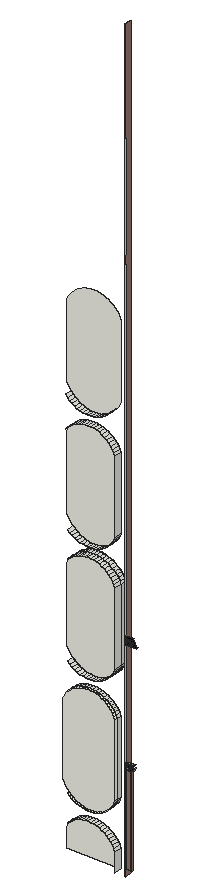
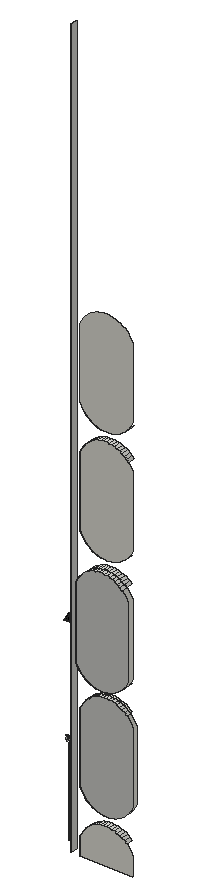
# SketchUp Ruby script. Lengths in inches.
U = 1.inch
M = Sketchup.active_model
def pt(a) = Geom::Point3d.new(a.map { |v| v * U })
def face(e, loops, mat)
  f = e.add_face(loops[0].map { |a| pt(a) })
  loops[1..].each { |l| e.add_face(l.map { |a| pt(a) }).erase! }
  f.material = f.back_material = mat if mat
  f
end
# faces: each face lists its corners as indices into pts; further lists are holes
def faces(e, pts, list, mat = nil) = list.each { |f| face(e, (f[0].is_a?(Array) ? f : [f]).map { |l| l.map { |i| pts[i] } }, mat) }
# xy, xz, yz: faces in a plane at the given z, y or x. An outline is a flat list of corners, or four numbers for a rectangle; further outlines are holes
def ring(l) = l.size == 4 ? [[l[0], l[1]], [l[2], l[1]], [l[2], l[3]], [l[0], l[3]]] : l.each_slice(2).to_a
def flat(e, list, mat, &to3) = list.each { |f| face(e, (f[0].is_a?(Array) ? f : [f]).map { |l| ring(l).map { |u, v| to3.(u, v) } }, mat) }
def xy(e, z, list, mat = nil) = flat(e, list, mat) { |x, y| [x, y, z] }
def xz(e, y, list, mat = nil) = flat(e, list, mat) { |x, z| [x, y, z] }
def yz(e, x, list, mat = nil) = flat(e, list, mat) { |y, z| [x, y, z] }
def lines(e, pts, list) = list.each { |a, b| e.add_line(pt(pts[a]), pt(pts[b])) }
# prism: a flat outline (further loops are holes) pulled along v
def prism(e, loops, v, mat = nil)
  f = face(e, loops, mat); d = Geom::Vector3d.new(v.map { |x| x * U })
  f.pushpull(f.normal.samedirection?(d) ? d.length : -d.length)
end
def box(e, o, s, mat = nil) = prism(e, [[o, [o[0] + s[0], o[1], o[2]], [o[0] + s[0], o[1] + s[1], o[2]], [o[0], o[1] + s[1], o[2]]]], [0, 0, s[2]], mat)
def at(x, y, z, deg = 0) = Geom::Transformation.translation(pt([x, y, z])) * Geom::Transformation.rotation(ORIGIN, Z_AXIS, deg.degrees)
def axes(o, x, y, z) = Geom::Transformation.new([*x, 0, *y, 0, *z, 0, *pt(o).to_a, 1])
def part(name) = M.definitions.add(name)
# library, detail: a bought-in or finely detailed component or shape, given as its bounding box
def library(name, o, s) = part(name).tap { |d| box(d.entities, o, s) }
def detail(e, o, s) = box(e.add_group.entities, o, s)
def put(e, d, t, mat = nil) = e.add_instance(d, t).tap { |i| i.material = mat if mat }
def group(e, t, mat = nil) = e.add_group.tap { |g| g.transformation = t; g.material = mat if mat }.entities
root = M.entities
M.materials.add("Tafisa-Gardenia-or-Gardenia-PM775-4K").color = [246, 245, 235]
M.materials.add("Tafisa-Terrarossa-PM780-4K").color = [148, 117, 107]
M.materials.add("Uniboard-L19-Putty-4K").color = [187, 181, 160]
M.materials.add("[Color M09]").color = [0, 0, 0]
xy(root,6.71,[[101.21,138,101.33,138.16]])
xy(root,16.52,[[101.21,138,101.33,138.16]])
xy(root,16.64,[[100.8125,138,101.11,138.16]])
xy(root,17.1,[[101.14,138,101.4,138.16]])
xy(root,17.16,[[100.67,138,100.85,138.16]])
xz(root,138,[[100.62,6.71,101.21,16.52]],"Tafisa-Terrarossa-PM780-4K")
xz(root,138,[[[100.62,16.52,100.93,17.21,100.62,17.2],[100.67,16.75,100.67,17.16,100.85,17.16]],[[100.62,16.52,101.33,16.52,100.93,17.21],[100.8125,16.64,100.94,16.9375,101.11,16.64]],[[101.33,16.52,101.58,17.24,100.93,17.21],[101.3,16.82,101.14,17.1,101.4,17.1]],[[100.62,28.8125,101.22,28.83,100.62,29.67],[100.74,28.9375,100.74,29.29,100.99,28.95]],[[101.22,28.83,101.42,29.64,100.62,29.67],[101.17,29.12,100.86,29.54,101.27,29.52]],
  [[101.22,28.83,101.82,28.85,101.42,29.64],[101.38,28.96,101.46,29.29,101.625,28.97]]],"[Color M09]")
xz(root,138.16,[[100.8125,16.64,101.11,16.64,100.94,16.9375],[100.67,16.75,100.85,17.16,100.67,17.16],[101.3,16.82,101.4,17.1,101.14,17.1]])
xz(root,138.16,[[101.21,6.71,101.33,16.52]],"Tafisa-Terrarossa-PM780-4K")
xz(root,138.16,[[100.74,28.9375,100.99,28.95,100.74,29.29],[101.38,28.96,101.625,28.97,101.46,29.29],[101.17,29.12,101.27,29.52,100.86,29.54]],"[Color M09]")
xz(root,138.25,[[96.53,11,96.85,11.02,97.16,11.0625,97.47,11.14,97.76,11.25,98.05,11.38,98.32,11.55,98.57,11.74,98.81,11.95,99.02,12.19,99.21,12.44,99.37,12.71,99.5,13,99.5,21,99.37,21.29,99.21,21.56,99.02,21.81,98.81,22.05,98.57,22.26,98.32,22.45,98.05,22.62,97.76,22.75,97.47,22.86,97.16,22.9375,96.85,22.98,96.53,23,96.22,22.98,95.9,22.9375,95.6,22.86,95.3,22.75,95.01,22.62,94.74,22.45,94.49,22.26,94.25,22.05,94.04,21.81,93.86,21.56,93.7,21.29,93.5625,21,93.5625,13,93.7,12.71,93.86,12.44,94.04,12.19,94.25,11.95,94.49,11.74,94.74,11.55,95.01,11.38,95.3,11.25,95.6,11.14,95.9,11.0625,96.22,11.02]],"Tafisa-Gardenia-or-Gardenia-PM775-4K")
xz(root,138.71,[[100.5,6,100.62,90]],"Tafisa-Gardenia-or-Gardenia-PM775-4K")
xz(root,138.79,[[96.53,11,96.85,11.02,97.16,11.0625,97.47,11.14,97.76,11.25,98.05,11.38,98.32,11.55,98.57,11.74,98.81,11.95,99.02,12.19,99.21,12.44,99.37,12.71,99.5,13,99.5,21,99.37,21.29,99.21,21.56,99.02,21.81,98.81,22.05,98.57,22.26,98.32,22.45,98.05,22.62,97.76,22.75,97.47,22.86,97.16,22.9375,96.85,22.98,96.53,23,96.22,22.98,95.9,22.9375,95.6,22.86,95.3,22.75,95.01,22.62,94.74,22.45,94.49,22.26,94.25,22.05,94.04,21.81,93.86,21.56,93.7,21.29,93.5625,21,93.5625,13,93.7,12.71,93.86,12.44,94.04,12.19,94.25,11.95,94.49,11.74,94.74,11.55,95.01,11.38,95.3,11.25,95.6,11.14,95.9,11.0625,96.22,11.02]])
xz(root,138.79,[[93.5625,6,99.5,6,99.5,8,99.37,8.29,99.21,8.56,99.02,8.81,98.81,9.05,98.57,9.26,98.32,9.45,98.05,9.62,97.76,9.75,97.47,9.86,97.16,9.9375,96.85,9.98,96.53,10,96.22,9.98,95.9,9.9375,95.6,9.86,95.3,9.75,95.01,9.62,94.74,9.45,94.49,9.26,94.25,9.05,94.04,8.81,93.86,8.56,93.7,8.29,93.5625,8],[96.53,24,96.85,24.02,97.16,24.0625,97.47,24.14,97.76,24.25,98.05,24.38,98.32,24.55,98.57,24.74,98.81,24.95,99.02,25.19,99.21,25.44,99.37,25.71,99.5,26,99.5,34,99.37,34.29,99.21,34.56,99.02,34.81,98.81,35.05,98.57,35.26,98.32,35.45,98.05,35.62,97.76,35.75,97.47,35.86,97.16,35.9375,96.85,35.98,96.53,36,96.22,35.98,95.9,35.9375,95.6,35.86,95.3,35.75,95.01,35.62,94.74,35.45,94.49,35.26,94.25,35.05,94.04,34.81,93.86,34.56,93.7,34.29,93.5625,34,93.5625,26,93.7,25.71,93.86,25.44,94.04,25.19,94.25,24.95,94.49,24.74,94.74,24.55,95.01,24.38,95.3,24.25,95.6,24.14,95.9,24.0625,96.22,24.02],[96.53,37,96.85,37.02,97.16,37.0625,97.47,37.14,97.76,37.25,98.05,37.38,98.32,37.55,98.57,37.74,98.81,37.95,99.02,38.19,99.21,38.44,99.37,38.71,99.5,39,99.5,47,99.37,47.29,99.21,47.56,99.02,47.81,98.81,48.05,98.57,48.26,98.32,48.45,98.05,48.62,97.76,48.75,97.47,48.86,97.16,48.9375,96.85,48.98,96.53,49,96.22,48.98,95.9,48.9375,95.6,48.86,95.3,48.75,95.01,48.62,94.74,48.45,94.49,48.26,94.25,48.05,94.04,47.81,93.86,47.56,93.7,47.29,93.5625,47,93.5625,39,93.7,38.71,93.86,38.44,94.04,38.19,94.25,37.95,94.49,37.74,94.74,37.55,95.01,37.38,95.3,37.25,95.6,37.14,95.9,37.0625,96.22,37.02],[96.53,50,96.85,50.02,97.16,50.0625,97.47,50.14,97.76,50.25,98.05,50.38,98.32,50.55,98.57,50.74,98.81,50.95,99.02,51.19,99.21,51.44,99.37,51.71,99.5,52,99.5,60,99.37,60.29,99.21,60.56,99.02,60.81,98.81,61.05,98.57,61.26,98.32,61.45,98.05,61.62,97.76,61.75,97.47,61.86,97.16,61.9375,96.85,61.98,96.53,62,96.22,61.98,95.9,61.9375,95.6,61.86,95.3,61.75,95.01,61.62,94.74,61.45,94.49,61.26,94.25,61.05,94.04,60.81,93.86,60.56,93.7,60.29,93.5625,60,93.5625,52,93.7,51.71,93.86,51.44,94.04,51.19,94.25,50.95,94.49,50.74,94.74,50.55,95.01,50.38,95.3,50.25,95.6,50.14,95.9,50.0625,96.22,50.02]],"Tafisa-Gardenia-or-Gardenia-PM775-4K")
xz(root,139.4375,[[96.53,24,96.85,24.02,97.16,24.0625,97.47,24.14,97.76,24.25,98.05,24.38,98.32,24.55,98.57,24.74,98.81,24.95,99.02,25.19,99.21,25.44,99.37,25.71,99.5,26,99.5,34,99.37,34.29,99.21,34.56,99.02,34.81,98.81,35.05,98.57,35.26,98.32,35.45,98.05,35.62,97.76,35.75,97.47,35.86,97.16,35.9375,96.85,35.98,96.53,36,96.22,35.98,95.9,35.9375,95.6,35.86,95.3,35.75,95.01,35.62,94.74,35.45,94.49,35.26,94.25,35.05,94.04,34.81,93.86,34.56,93.7,34.29,93.5625,34,93.5625,26,93.7,25.71,93.86,25.44,94.04,25.19,94.25,24.95,94.49,24.74,94.74,24.55,95.01,24.38,95.3,24.25,95.6,24.14,95.9,24.0625,96.22,24.02]])
yz(root,99.5,[[138,6,138.79,8],[138.25,13,138.79,21],[138,26,138.79,34],[138.79,26,139.4375,34],[138,39,138.79,47]])
yz(root,99.5,[[138,13,138.25,21]],"Tafisa-Gardenia-or-Gardenia-PM775-4K")
yz(root,100.5,[[138,6,138.71,90]])
yz(root,100.62,[[138,6,138,17.2,138.16,17.2,138.16,28.8125,138,28.8125,138,29.67,138.16,29.67,138.16,66.38,138,66.38,138,67.1875,138.16,67.1875,138.16,78.8,138,78.8,138,90,138.71,90,138.71,6]],"Tafisa-Terrarossa-PM780-4K")
yz(root,100.67,[[138,16.75,138.16,17.16]])
yz(root,100.74,[[138,28.9375,138.16,29.29]],"[Color M09]")
yz(root,101.21,[[138,6.71,138.16,16.52]],"Tafisa-Terrarossa-PM780-4K")
yz(root,101.33,[[138,6.71,138.16,16.52]],"Tafisa-Terrarossa-PM780-4K")
p = [[99.37,138.79,8.29],[99.5,138.79,8],[99.5,138,8],[99.37,138,8.29],[99.21,138.79,8.56],[99.21,138,8.56],
  [99.02,138.79,8.81],[99.02,138,8.81],[98.81,138.79,9.05],[98.81,138,9.05],[94.25,138.79,9.05],[94.49,138.79,9.26],
  [94.49,138,9.26],[94.25,138,9.05],[98.57,138.79,9.26],[98.57,138,9.26],[94.74,138.79,9.45],[94.74,138,9.45],
  [98.32,138.79,9.45],[98.32,138,9.45],[95.01,138.79,9.62],[95.01,138,9.62],[98.05,138.79,9.62],[98.05,138,9.62],
  [95.3,138.79,9.75],[95.3,138,9.75],[97.76,138.79,9.75],[97.76,138,9.75],[95.6,138.79,9.86],[95.6,138,9.86],
  [97.47,138.79,9.86],[97.47,138,9.86],[95.9,138.79,9.9375],[95.9,138,9.9375],[96.22,138.79,9.98],[96.22,138,9.98],
  [96.85,138.79,9.98],[97.16,138.79,9.9375],[97.16,138,9.9375],[96.85,138,9.98],[96.53,138.79,10],[96.53,138,10],
  [95.9,138,11.0625],[96.22,138,11.02],[96.22,138.25,11.02],[95.9,138.25,11.0625],[96.53,138,11],[96.53,138.25,11],
  [96.85,138,11.02],[96.85,138.25,11.02],[97.16,138,11.0625],[97.16,138.25,11.0625],[96.22,138.79,11.02],[95.9,138.79,11.0625],
  [96.53,138.79,11],[96.85,138.79,11.02],[97.16,138.79,11.0625],[95.3,138,11.25],[95.6,138,11.14],[95.6,138.25,11.14],
  [95.3,138.25,11.25],[97.47,138,11.14],[97.47,138.25,11.14],[97.76,138,11.25],[97.76,138.25,11.25],[95.6,138.79,11.14],
  [95.3,138.79,11.25],[97.47,138.79,11.14],[97.76,138.79,11.25],[95.01,138,11.38],[95.01,138.25,11.38],[98.05,138,11.38],
  [98.05,138.25,11.38],[95.01,138.79,11.38],[98.05,138.79,11.38],[94.74,138,11.55],[94.74,138.25,11.55],[98.32,138,11.55],
  [98.32,138.25,11.55],[94.74,138.79,11.55],[98.32,138.79,11.55],[94.49,138,11.74],[94.49,138.25,11.74],[98.57,138,11.74],
  [98.57,138.25,11.74],[94.49,138.79,11.74],[98.57,138.79,11.74],[94.25,138,11.95],[94.25,138.25,11.95],[98.81,138,11.95],
  [98.81,138.25,11.95],[94.25,138.79,11.95],[98.81,138.79,11.95],[99.02,138,12.19],[99.02,138.25,12.19],[99.02,138.79,12.19],
  [99.21,138,12.44],[99.21,138.25,12.44],[99.21,138.79,12.44],[99.37,138,12.71],[99.37,138.25,12.71],[99.37,138.79,12.71],
  [99.5,138,13],[99.5,138.25,13],[99.5,138.79,13],[100.94,138,16.9375],[100.8125,138,16.64],[100.8125,138.16,16.64],
  [100.94,138.16,16.9375],[101.11,138,16.64],[101.11,138.16,16.64],[101.61,138,16.93],[101.51,138,16.65],[101.51,138.16,16.65],
  [101.61,138.16,16.93],[100.67,138,16.75],[100.85,138,17.16],[100.85,138.16,17.16],[100.67,138.16,16.75],[101.14,138,17.1],
  [101.3,138,16.82],[101.3,138.16,16.82],[101.14,138.16,17.1],[101.4,138,17.1],[101.4,138.16,17.1],[100.62,138,17.2],
  [100.93,138,17.21],[100.93,138.16,17.21],[100.62,138.16,17.2],[101.58,138,17.24],[101.58,138.16,17.24],[99.5,138,21],
  [99.37,138,21.29],[99.37,138.25,21.29],[99.5,138.25,21],[99.37,138.79,21.29],[99.5,138.79,21],[99.21,138,21.56],
  [99.21,138.25,21.56],[99.21,138.79,21.56],[99.02,138,21.81],[99.02,138.25,21.81],[99.02,138.79,21.81],[98.81,138,22.05],
  [98.81,138.25,22.05],[98.81,138.79,22.05],[94.49,138,22.26],[94.25,138,22.05],[94.25,138.25,22.05],[94.49,138.25,22.26],
  [98.57,138,22.26],[98.57,138.25,22.26],[94.25,138.79,22.05],[94.49,138.79,22.26],[98.57,138.79,22.26],[94.74,138,22.45],
  [94.74,138.25,22.45],[98.32,138,22.45],[98.32,138.25,22.45],[94.74,138.79,22.45],[98.32,138.79,22.45],[95.01,138,22.62],
  [95.01,138.25,22.62],[98.05,138,22.62],[98.05,138.25,22.62],[95.01,138.79,22.62],[98.05,138.79,22.62],[95.3,138,22.75],
  [95.3,138.25,22.75],[97.76,138,22.75],[97.76,138.25,22.75],[95.3,138.79,22.75],[97.76,138.79,22.75],[95.6,138,22.86],
  [95.6,138.25,22.86],[97.47,138,22.86],[97.47,138.25,22.86],[95.6,138.79,22.86],[97.47,138.79,22.86],[95.9,138,22.9375],
  [95.9,138.25,22.9375],[96.22,138,22.98],[96.22,138.25,22.98],[97.16,138,22.9375],[96.85,138,22.98],[96.85,138.25,22.98],
  [97.16,138.25,22.9375],[95.9,138.79,22.9375],[96.22,138.79,22.98],[96.85,138.79,22.98],[97.16,138.79,22.9375],[96.53,138,23],
  [96.53,138.25,23],[96.53,138.79,23],[96.22,138.79,24.02],[95.9,138.79,24.0625],[95.9,138,24.0625],[96.22,138,24.02],
  [96.53,138.79,24],[96.53,138,24],[96.85,138.79,24.02],[96.85,138,24.02],[97.16,138.79,24.0625],[97.16,138,24.0625],
  [95.9,139.4375,24.0625],[96.22,139.4375,24.02],[96.53,139.4375,24],[96.85,139.4375,24.02],[97.16,139.4375,24.0625],[95.6,138.79,24.14],
  [95.3,138.79,24.25],[95.3,138,24.25],[95.6,138,24.14],[97.47,138.79,24.14],[97.47,138,24.14],[97.76,138.79,24.25],
  [97.76,138,24.25],[95.3,139.4375,24.25],[95.6,139.4375,24.14],[97.47,139.4375,24.14],[97.76,139.4375,24.25],[95.01,138.79,24.38],
  [95.01,138,24.38],[98.05,138.79,24.38],[98.05,138,24.38],[95.01,139.4375,24.38],[98.05,139.4375,24.38],[94.74,138.79,24.55],
  [94.74,138,24.55],[98.32,138.79,24.55],[98.32,138,24.55],[94.74,139.4375,24.55],[98.32,139.4375,24.55],[94.49,138.79,24.74],
  [94.49,138,24.74],[98.57,138.79,24.74],[98.57,138,24.74],[94.49,139.4375,24.74],[98.57,139.4375,24.74],[94.25,138.79,24.95],
  [94.25,138,24.95],[98.81,138.79,24.95],[98.81,138,24.95],[94.25,139.4375,24.95],[98.81,139.4375,24.95],[99.02,138.79,25.19],
  [99.02,138,25.19],[99.02,139.4375,25.19],[99.21,138.79,25.44],[99.21,138,25.44],[99.21,139.4375,25.44],[99.37,138.79,25.71],
  [99.37,138,25.71],[99.37,139.4375,25.71],[99.5,138.79,26],[99.5,138,26],[99.5,139.4375,26],[101.22,138,28.83],
  [100.62,138,28.8125],[100.62,138.16,28.8125],[101.22,138.16,28.83],[101.82,138,28.85],[101.82,138.16,28.85],[100.74,138,28.9375],
  [100.99,138,28.95],[100.99,138.16,28.95],[100.74,138.16,28.9375],[100.74,138,29.29],[100.74,138.16,29.29],[101.46,138,29.29],
  [101.38,138,28.96],[101.38,138.16,28.96],[101.46,138.16,29.29],[101.625,138,28.97],[101.625,138.16,28.97],[100.86,138,29.54],
  [101.17,138,29.12],[101.17,138.16,29.12],[100.86,138.16,29.54],[101.27,138,29.52],[101.27,138.16,29.52],[100.62,138,29.67],
  [101.42,138,29.64],[101.42,138.16,29.64],[100.62,138.16,29.67],[99.37,138.79,34.29],[99.5,138.79,34],[99.5,138,34],
  [99.37,138,34.29],[99.5,139.4375,34],[99.37,139.4375,34.29],[99.21,138.79,34.56],[99.21,138,34.56],[99.21,139.4375,34.56],
  [99.02,138.79,34.81],[99.02,138,34.81],[99.02,139.4375,34.81],[98.81,138.79,35.05],[98.81,138,35.05],[98.81,139.4375,35.05],
  [94.25,138.79,35.05],[94.49,138.79,35.26],[94.49,138,35.26],[94.25,138,35.05],[98.57,138.79,35.26],[98.57,138,35.26],
  [94.49,139.4375,35.26],[94.25,139.4375,35.05],[98.57,139.4375,35.26],[94.74,138.79,35.45],[94.74,138,35.45],[98.32,138.79,35.45],
  [98.32,138,35.45],[94.74,139.4375,35.45],[98.32,139.4375,35.45],[95.01,138.79,35.62],[95.01,138,35.62],[98.05,138.79,35.62],
  [98.05,138,35.62],[95.01,139.4375,35.62],[98.05,139.4375,35.62],[95.3,138.79,35.75],[95.3,138,35.75],[97.76,138.79,35.75],
  [97.76,138,35.75],[95.3,139.4375,35.75],[97.76,139.4375,35.75],[95.6,138.79,35.86],[95.6,138,35.86],[97.47,138.79,35.86],
  [97.47,138,35.86],[95.6,139.4375,35.86],[97.47,139.4375,35.86],[95.9,138.79,35.9375],[95.9,138,35.9375],[96.22,138.79,35.98],
  [96.22,138,35.98],[96.85,138.79,35.98],[97.16,138.79,35.9375],[97.16,138,35.9375],[96.85,138,35.98],[95.9,139.4375,35.9375],
  [96.22,139.4375,35.98],[97.16,139.4375,35.9375],[96.85,139.4375,35.98],[96.53,138.79,36],[96.53,138,36],[96.53,139.4375,36],
  [96.22,138.79,37.02],[95.9,138.79,37.0625],[95.9,138,37.0625],[96.22,138,37.02],[96.53,138.79,37],[96.53,138,37],
  [96.85,138.79,37.02],[96.85,138,37.02],[97.16,138.79,37.0625],[97.16,138,37.0625],[95.6,138.79,37.14],[95.3,138.79,37.25],
  [95.3,138,37.25],[95.6,138,37.14],[97.47,138.79,37.14],[97.47,138,37.14],[97.76,138.79,37.25],[97.76,138,37.25],
  [95.01,138.79,37.38],[95.01,138,37.38],[98.05,138.79,37.38],[98.05,138,37.38],[94.74,138.79,37.55],[94.74,138,37.55],
  [98.32,138.79,37.55],[98.32,138,37.55],[94.49,138.79,37.74],[94.49,138,37.74],[98.57,138.79,37.74],[98.57,138,37.74],
  [94.25,138.79,37.95],[94.25,138,37.95],[98.81,138.79,37.95],[98.81,138,37.95],[99.02,138.79,38.19],[99.02,138,38.19],
  [99.21,138.79,38.44],[99.21,138,38.44],[99.37,138.79,38.71],[99.37,138,38.71],[99.5,138.79,39],[99.5,138,39],
  [99.37,138.79,47.29],[99.5,138.79,47],[99.5,138,47],[99.37,138,47.29],[99.21,138.79,47.56],[99.21,138,47.56],
  [99.02,138.79,47.81],[99.02,138,47.81],[94.04,138.79,47.81],[94.25,138.79,48.05],[94.25,138,48.05],[94.04,138,47.81],
  [98.81,138.79,48.05],[98.81,138,48.05],[94.49,138.79,48.26],[94.49,138,48.26],[98.57,138.79,48.26],[98.57,138,48.26],
  [94.74,138.79,48.45],[94.74,138,48.45],[98.32,138.79,48.45],[98.32,138,48.45],[95.01,138.79,48.62],[95.01,138,48.62],
  [98.05,138.79,48.62],[98.05,138,48.62],[95.3,138.79,48.75],[95.3,138,48.75],[97.76,138.79,48.75],[97.76,138,48.75],
  [95.6,138.79,48.86],[95.6,138,48.86],[97.47,138.79,48.86],[97.47,138,48.86],[95.9,138.79,48.9375],[95.9,138,48.9375],
  [96.22,138.79,48.98],[96.22,138,48.98],[96.85,138.79,48.98],[97.16,138.79,48.9375],[97.16,138,48.9375],[96.85,138,48.98],
  [96.53,138.79,49],[96.53,138,49],[96.22,138.79,50.02],[95.9,138.79,50.0625],[95.9,138,50.0625],[96.22,138,50.02],
  [96.53,138.79,50],[96.53,138,50],[96.85,138.79,50.02],[96.85,138,50.02],[97.16,138.79,50.0625],[97.16,138,50.0625],
  [95.6,138.79,50.14],[95.3,138.79,50.25],[95.3,138,50.25],[95.6,138,50.14],[97.47,138.79,50.14],[97.47,138,50.14],
  [97.76,138.79,50.25],[97.76,138,50.25],[95.01,138.79,50.38],[95.01,138,50.38],[98.05,138.79,50.38],[98.05,138,50.38],
  [94.74,138.79,50.55],[94.74,138,50.55],[98.32,138.79,50.55],[98.32,138,50.55],[94.49,138.79,50.74],[94.49,138,50.74],
  [98.57,138.79,50.74],[98.57,138,50.74],[94.25,138.79,50.95],[94.25,138,50.95],[98.81,138.79,50.95],[98.81,138,50.95],
  [94.04,138.79,51.19],[94.04,138,51.19],[99.02,138.79,51.19],[99.02,138,51.19],[100.5,138,28.82]]
faces(root,p,[[0,1,2,3],[4,0,3,5],[6,4,5,7],[8,6,7,9],[10,11,12,13],[14,8,9,15],[11,16,17,12],[18,14,15,19],
  [16,20,21,17],[22,18,19,23],[20,24,25,21],[26,22,23,27],[24,28,29,25],[30,26,27,31],[28,32,33,29],[32,34,35,33],
  [36,37,38,39],[37,30,31,38],[34,40,41,35],[40,36,39,41],[52,53,45,44],[54,52,44,47],[55,54,47,49],[56,55,49,51],
  [65,66,60,59],[53,65,59,45],[67,56,51,62],[68,67,62,64],[66,73,70,60],[74,68,64,72],[73,79,76,70],[80,74,72,78],
  [79,85,82,76],[86,80,78,84],[85,91,88,82],[92,86,84,90],[95,92,90,94],[98,95,94,97],[101,98,97,100],[104,101,100,103],
  [105,106,107,108],[109,105,108,110],[111,112,113,114],[115,116,117,118],[119,120,121,122],[120,123,124,121],[135,136,134,133],[139,135,133,138],
  [142,139,138,141],[145,142,141,144],[152,153,149,148],[154,145,144,151],[153,159,156,149],[160,154,151,158],[159,165,162,156],[166,160,158,164],
  [165,171,168,162],[172,166,164,170],[171,177,174,168],[178,172,170,176],[177,187,180,174],[187,188,182,180],[189,190,186,185],[190,178,176,186],
  [188,193,192,182],[193,189,185,192],[194,195,196,197],[198,194,197,199],[200,198,199,201],[202,200,201,203],[204,195,194,205],[205,194,198,206],
  [206,198,200,207],[207,200,202,208],[209,210,211,212],[195,209,212,196],[213,202,203,214],[215,213,214,216],[217,210,209,218],[218,209,195,204],
  [208,202,213,219],[219,213,215,220],[210,221,222,211],[223,215,216,224],[225,221,210,217],[220,215,223,226],[221,227,228,222],[229,223,224,230],
  [231,227,221,225],[226,223,229,232],[227,233,234,228],[235,229,230,236],[237,233,227,231],[232,229,235,238],[233,239,240,234],[241,235,236,242],
  [243,239,233,237],[238,235,241,244],[245,241,242,246],[244,241,245,247],[248,245,246,249],[247,245,248,250],[251,248,249,252],[250,248,251,253],
  [254,251,252,255],[253,251,254,256],[285,286,287,288],[289,286,285,290],[291,285,288,292],[290,285,291,293],[294,291,292,295],[293,291,294,296],
  [297,294,295,298],[296,294,297,299],[300,301,302,303],[304,297,298,305],[306,301,300,307],[299,297,304,308],[301,309,310,302],[311,304,305,312],
  [313,309,301,306],[308,304,311,314],[309,315,316,310],[317,311,312,318],[319,315,309,313],[314,311,317,320],[315,321,322,316],[323,317,318,324],
  [325,321,315,319],[320,317,323,326],[321,327,328,322],[329,323,324,330],[331,327,321,325],[326,323,329,332],[327,333,334,328],[333,335,336,334],
  [337,338,339,340],[338,329,330,339],[341,333,327,331],[342,335,333,341],[343,338,337,344],[332,329,338,343],[335,345,346,336],[345,337,340,346],
  [347,345,335,342],[344,337,345,347],[348,349,350,351],[352,348,351,353],[354,352,353,355],[356,354,355,357],[358,359,360,361],[349,358,361,350],
  [362,356,357,363],[364,362,363,365],[359,366,367,360],[368,364,365,369],[366,370,371,367],[372,368,369,373],[370,374,375,371],[376,372,373,377],
  [374,378,379,375],[380,376,377,381],[382,380,381,383],[384,382,383,385],[386,384,385,387],[388,386,387,389],[390,391,392,393],[394,390,393,395],
  [396,394,395,397],[398,399,400,401],[402,396,397,403],[399,404,405,400],[406,402,403,407],[404,408,409,405],[410,406,407,411],[408,412,413,409],
  [414,410,411,415],[412,416,417,413],[418,414,415,419],[416,420,421,417],[422,418,419,423],[420,424,425,421],[424,426,427,425],[428,429,430,431],
  [429,422,423,430],[426,432,433,427],[432,428,431,433],[434,435,436,437],[438,434,437,439],[440,438,439,441],[442,440,441,443],[444,445,446,447],
  [435,444,447,436],[448,442,443,449],[450,448,449,451],[445,452,453,446],[454,450,451,455],[452,456,457,453],[458,454,455,459],[456,460,461,457],
  [462,458,459,463],[460,464,465,461],[466,462,463,467],[464,468,469,465],[470,466,467,471]])
faces(root,p,[[42,43,44,45],[43,46,47,44],[46,48,49,47],[48,50,51,49],[57,58,59,60],[58,42,45,59],[50,61,62,51],[61,63,64,62],
  [69,57,60,70],[63,71,72,64],[75,69,70,76],[71,77,78,72],[81,75,76,82],[77,83,84,78],[87,81,82,88],[83,89,90,84],
  [89,93,94,90],[93,96,97,94],[96,99,100,97],[99,102,103,100],[131,132,133,134],[132,137,138,133],[137,140,141,138],[140,143,144,141],
  [146,147,148,149],[143,150,151,144],[155,146,149,156],[150,157,158,151],[161,155,156,162],[157,163,164,158],[167,161,162,168],[163,169,170,164],
  [173,167,168,174],[169,175,176,170],[179,173,174,180],[181,179,180,182],[183,184,185,186],[175,183,186,176],[191,181,182,192],[184,191,192,185]],"Tafisa-Gardenia-or-Gardenia-PM775-4K")
faces(root,p,[[125,126,127,128],[126,129,130,127]],"Uniboard-L19-Putty-4K")
faces(root,p,[[257,258,259,260],[261,257,260,262],[263,264,265,266],[264,267,268,265],[269,270,271,272],[270,273,274,271],[273,269,272,274],[275,276,277,278],
  [276,279,280,277],[279,275,278,280],[281,282,283,284]],"[Color M09]")
lines(root,p,[[258,472]])
